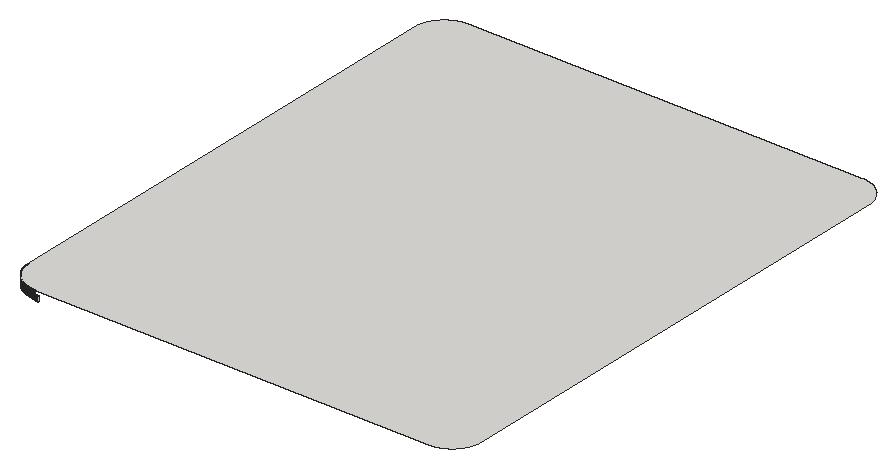
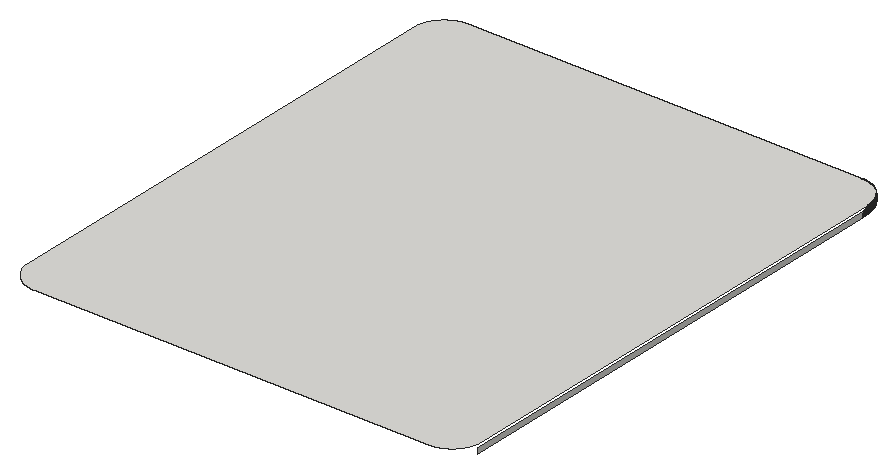
# SketchUp Ruby script. Lengths in inches.
U = 1.inch
M = Sketchup.active_model
def pt(a) = Geom::Point3d.new(a.map { |v| v * U })
def face(e, loops, mat)
  f = e.add_face(loops[0].map { |a| pt(a) })
  loops[1..].each { |l| e.add_face(l.map { |a| pt(a) }).erase! }
  f.material = f.back_material = mat if mat
  f
end
# faces: each face lists its corners as indices into pts; further lists are holes
def faces(e, pts, list, mat = nil) = list.each { |f| face(e, (f[0].is_a?(Array) ? f : [f]).map { |l| l.map { |i| pts[i] } }, mat) }
# xy, xz, yz: faces in a plane at the given z, y or x. An outline is a flat list of corners, or four numbers for a rectangle; further outlines are holes
def ring(l) = l.size == 4 ? [[l[0], l[1]], [l[2], l[1]], [l[2], l[3]], [l[0], l[3]]] : l.each_slice(2).to_a
def flat(e, list, mat, &to3) = list.each { |f| face(e, (f[0].is_a?(Array) ? f : [f]).map { |l| ring(l).map { |u, v| to3.(u, v) } }, mat) }
def xy(e, z, list, mat = nil) = flat(e, list, mat) { |x, y| [x, y, z] }
def xz(e, y, list, mat = nil) = flat(e, list, mat) { |x, z| [x, y, z] }
def yz(e, x, list, mat = nil) = flat(e, list, mat) { |y, z| [x, y, z] }
def lines(e, pts, list) = list.each { |a, b| e.add_line(pt(pts[a]), pt(pts[b])) }
# prism: a flat outline (further loops are holes) pulled along v
def prism(e, loops, v, mat = nil)
  f = face(e, loops, mat); d = Geom::Vector3d.new(v.map { |x| x * U })
  f.pushpull(f.normal.samedirection?(d) ? d.length : -d.length)
end
def box(e, o, s, mat = nil) = prism(e, [[o, [o[0] + s[0], o[1], o[2]], [o[0] + s[0], o[1] + s[1], o[2]], [o[0], o[1] + s[1], o[2]]]], [0, 0, s[2]], mat)
def at(x, y, z, deg = 0) = Geom::Transformation.translation(pt([x, y, z])) * Geom::Transformation.rotation(ORIGIN, Z_AXIS, deg.degrees)
def axes(o, x, y, z) = Geom::Transformation.new([*x, 0, *y, 0, *z, 0, *pt(o).to_a, 1])
def part(name) = M.definitions.add(name)
# library, detail: a bought-in or finely detailed component or shape, given as its bounding box
def library(name, o, s) = part(name).tap { |d| box(d.entities, o, s) }
def detail(e, o, s) = box(e.add_group.entities, o, s)
def put(e, d, t, mat = nil) = e.add_instance(d, t).tap { |i| i.material = mat if mat }
def group(e, t, mat = nil) = e.add_group.tap { |g| g.transformation = t; g.material = mat if mat }.entities
root = M.entities
M.materials.add("[Formica Graystone]").color = [224, 223, 219]
xy(root,427.82,[[17.6875,229,174.3125,229,174.47,229.01,174.63,229.02,174.78,229.03,175.1,229.05,175.25,229.07,175.41,229.08,175.57,229.1,175.72,229.125,175.88,229.15,176.03,229.17,176.1875,229.2,176.34,229.23,176.49,229.26,176.65,229.3,176.8,229.33,176.95,229.37,177.11,229.41,177.41,229.49,177.86,229.64,178.01,229.6875,178.15,229.74,178.3,229.8,178.45,229.85,178.59,229.91,178.74,229.97,178.88,230.04,179.02,230.1,179.17,230.17,179.73,230.45,179.86,230.53,180,230.61,180.14,230.6875,180.27,230.77,180.4,230.85,180.54,230.9375,180.67,231.02,180.93,231.2,181.05,231.29,181.18,231.38,181.31,231.48,181.43,231.58,181.55,231.67,181.67,231.77,181.91,231.98,182.03,232.08,182.15,232.1875,182.26,232.3,182.375,232.4,182.49,232.51,182.6,232.625,182.7,232.74,182.8125,232.85,182.92,232.97,183.02,233.09,183.23,233.33,183.33,233.45,183.42,233.57,183.52,233.69,183.62,233.82,183.71,233.95,183.8,234.07,183.98,234.33,184.0625,234.46,184.15,234.6,184.23,234.73,184.3125,234.86,184.39,235,184.47,235.14,184.55,235.27,184.83,235.83,184.9,235.98,184.96,236.12,185.03,236.26,185.09,236.41,185.15,236.55,185.2,236.7,185.26,236.85,185.3125,236.99,185.36,237.14,185.51,237.59,185.59,237.89,185.63,238.05,185.67,238.2,185.7,238.35,185.74,238.51,185.77,238.66,185.8,238.8125,185.83,238.97,185.85,239.12,185.875,239.28,185.9,239.43,185.92,239.59,185.93,239.75,185.95,239.9,185.97,240.22,185.98,240.37,185.99,240.53,186,240.6875,186,432.3125,185.99,432.47,185.98,432.63,185.97,432.78,185.95,433.1,185.93,433.25,185.92,433.41,185.9,433.57,185.875,433.72,185.85,433.88,185.83,434.03,185.8,434.1875,185.77,434.34,185.74,434.49,185.7,434.65,185.67,434.8,185.63,434.95,185.59,435.11,185.51,435.41,185.36,435.86,185.3125,436.01,185.26,436.15,185.2,436.3,185.15,436.45,185.09,436.59,185.03,436.74,184.96,436.88,184.9,437.02,184.83,437.17,184.55,437.73,184.47,437.86,184.39,438,184.3125,438.14,184.23,438.27,184.15,438.4,184.0625,438.54,183.98,438.67,183.8,438.93,183.71,439.05,183.62,439.18,183.52,439.31,183.42,439.43,183.33,439.55,183.23,439.67,183.02,439.91,182.92,440.03,182.8125,440.15,182.7,440.26,182.6,440.375,182.49,440.49,182.375,440.6,182.26,440.7,182.15,440.8125,182.03,440.92,181.91,441.02,181.67,441.23,181.55,441.33,181.43,441.42,181.31,441.52,181.18,441.62,181.05,441.71,180.93,441.8,180.67,441.98,180.54,442.0625,180.4,442.15,180.27,442.23,180.14,442.3125,180,442.39,179.86,442.47,179.73,442.55,179.17,442.83,179.02,442.9,178.88,442.96,178.74,443.03,178.59,443.09,178.45,443.15,178.3,443.2,178.15,443.26,178.01,443.3125,177.86,443.36,177.41,443.51,177.11,443.59,176.95,443.63,176.8,443.67,176.65,443.7,176.49,443.74,176.34,443.77,176.1875,443.8,176.03,443.83,175.88,443.85,175.72,443.875,175.57,443.9,175.41,443.92,175.25,443.93,175.1,443.95,174.78,443.97,174.63,443.98,174.47,443.99,174.3125,444,17.6875,444,17.53,443.99,17.37,443.98,17.22,443.97,16.9,443.95,16.75,443.93,16.59,443.92,16.43,443.9,16.28,443.875,16.12,443.85,15.97,443.83,15.8125,443.8,15.66,443.77,15.51,443.74,15.35,443.7,15.2,443.67,15.05,443.63,14.89,443.59,14.59,443.51,14.14,443.36,13.99,443.3125,13.85,443.26,13.7,443.2,13.55,443.15,13.41,443.09,13.26,443.03,13.12,442.96,12.98,442.9,12.83,442.83,12.27,442.55,12.14,442.47,12,442.39,11.86,442.3125,11.73,442.23,11.6,442.15,11.46,442.0625,11.33,441.98,11.07,441.8,10.95,441.71,10.82,441.62,10.69,441.52,10.57,441.42,10.45,441.33,10.33,441.23,10.09,441.02,9.97,440.92,9.85,440.8125,9.74,440.7,9.625,440.6,9.51,440.49,9.4,440.375,9.3,440.26,9.1875,440.15,9.08,440.03,8.98,439.91,8.77,439.67,8.67,439.55,8.58,439.43,8.48,439.31,8.38,439.18,8.29,439.05,8.2,438.93,8.02,438.67,7.9375,438.54,7.85,438.4,7.77,438.27,7.6875,438.14,7.61,438,7.53,437.86,7.45,437.73,7.17,437.17,7.1,437.02,7.04,436.88,6.97,436.74,6.91,436.59,6.85,436.45,6.8,436.3,6.74,436.15,6.6875,436.01,6.64,435.86,6.49,435.41,6.41,435.11,6.37,434.95,6.33,434.8,6.3,434.65,6.26,434.49,6.23,434.34,6.2,434.1875,6.17,434.03,6.15,433.88,6.125,433.72,6.1,433.57,6.08,433.41,6.07,433.25,6.05,433.1,6.03,432.78,6.02,432.63,6.01,432.47,6,432.3125,6,240.6875,6.01,240.53,6.02,240.37,6.03,240.22,6.05,239.9,6.07,239.75,6.08,239.59,6.1,239.43,6.125,239.28,6.15,239.12,6.17,238.97,6.2,238.8125,6.23,238.66,6.26,238.51,6.3,238.35,6.33,238.2,6.37,238.05,6.41,237.89,6.49,237.59,6.64,237.14,6.6875,236.99,6.74,236.85,6.8,236.7,6.85,236.55,6.91,236.41,6.97,236.26,7.04,236.12,7.1,235.98,7.17,235.83,7.45,235.27,7.53,235.14,7.61,235,7.6875,234.86,7.77,234.73,7.85,234.6,7.9375,234.46,8.02,234.33,8.2,234.07,8.29,233.95,8.38,233.82,8.48,233.69,8.58,233.57,8.67,233.45,8.77,233.33,8.98,233.09,9.08,232.97,9.1875,232.85,9.3,232.74,9.4,232.625,9.51,232.51,9.625,232.4,9.74,232.3,9.85,232.1875,9.97,232.08,10.09,231.98,10.33,231.77,10.45,231.67,10.57,231.58,10.69,231.48,10.82,231.38,10.95,231.29,11.07,231.2,11.33,231.02,11.46,230.9375,11.6,230.85,11.73,230.77,11.86,230.6875,12,230.61,12.14,230.53,12.27,230.45,12.83,230.17,12.98,230.1,13.12,230.04,13.26,229.97,13.41,229.91,13.55,229.85,13.7,229.8,13.85,229.74,13.99,229.6875,14.14,229.64,14.59,229.49,14.89,229.41,15.05,229.37,15.2,229.33,15.35,229.3,15.51,229.26,15.66,229.23,15.8125,229.2,15.97,229.17,16.12,229.15,16.28,229.125,16.43,229.1,16.59,229.08,16.75,229.07,16.9,229.05,17.22,229.03,17.37,229.02,17.53,229.01]],"[Formica Graystone]")
xz(root,229,[[17.6875,424.82,17.84,427.82],[17.84,424.82,18,427.82]],"[Formica Graystone]")
xz(root,231,[[17.74,422.82,17.87,424.82],[17.87,422.82,18,424.82]],"[Formica Graystone]")
xz(root,231.01,[[17.48,422.82,17.61,424.82]],"[Formica Graystone]")
yz(root,6,[[240.6875,424.82,240.84,427.82],[240.84,424.82,241,427.82]],"[Formica Graystone]")
yz(root,8,[[240.74,422.82,240.87,424.82],[240.87,422.82,241,424.82],[241,422.82,432,424.82]],"[Formica Graystone]")
yz(root,8.01,[[240.48,422.82,240.61,424.82]],"[Formica Graystone]")
p = [[17.08,231.04,422.82],[17.08,231.04,424.82],[16.95,231.05,424.82],[16.95,231.05,422.82],[17.22,231.03,422.82],[17.22,231.03,424.82],
  [17.35,231.02,422.82],[17.35,231.02,424.82],[17.48,231.01,422.82],[17.48,231.01,424.82],[17.74,231,422.82],[17.74,231,424.82],
  [17.61,231.01,424.82],[17.61,231.01,422.82],[16.31,231.14,422.82],[16.31,231.14,424.82],[16.18,231.17,424.82],[16.18,231.17,422.82],
  [16.4375,231.125,422.82],[16.4375,231.125,424.82],[16.57,231.1,422.82],[16.57,231.1,424.82],[16.69,231.09,422.82],[16.69,231.09,424.82],
  [16.82,231.07,422.82],[16.82,231.07,424.82],[15.79,231.25,422.82],[15.79,231.25,424.82],[15.67,231.28,424.82],[15.67,231.28,422.82],
  [15.92,231.22,422.82],[15.92,231.22,424.82],[16.05,231.19,422.82],[16.05,231.19,424.82],[15.41,231.34,422.82],[15.41,231.34,424.82],
  [15.29,231.375,424.82],[15.29,231.375,422.82],[15.54,231.31,422.82],[15.54,231.31,424.82],[15.03,231.45,422.82],[15.03,231.45,424.82],
  [14.91,231.49,424.82],[14.91,231.49,422.82],[15.16,231.41,422.82],[15.16,231.41,424.82],[14.79,231.53,422.82],[14.79,231.53,424.82],
  [14.66,231.57,424.82],[14.66,231.57,422.82],[14.54,231.62,422.82],[14.54,231.62,424.82],[14.42,231.66,424.82],[14.42,231.66,422.82],
  [14.29,231.71,422.82],[14.29,231.71,424.82],[14.17,231.76,424.82],[14.17,231.76,422.82],[14.05,231.8125,422.82],[14.05,231.8125,424.82],
  [13.93,231.86,424.82],[13.93,231.86,422.82],[13.8125,231.92,422.82],[13.8125,231.92,424.82],[13.69,231.97,424.82],[13.69,231.97,422.82],
  [13.58,232.03,422.82],[13.58,232.03,424.82],[13.46,232.09,424.82],[13.46,232.09,422.82],[13.34,232.15,424.82],[13.34,232.15,422.82],
  [13.23,232.21,422.82],[13.23,232.21,424.82],[13.11,232.28,424.82],[13.11,232.28,422.82],[13,232.34,422.82],[13,232.34,424.82],
  [12.89,232.41,424.82],[12.89,232.41,422.82],[12.78,232.47,424.82],[12.78,232.47,422.82],[12.66,232.54,422.82],[12.66,232.54,424.82],
  [12.55,232.61,424.82],[12.55,232.61,422.82],[12.44,232.69,424.82],[12.44,232.69,422.82],[12.34,232.76,424.82],[12.34,232.76,422.82],
  [12.23,232.83,422.82],[12.23,232.83,424.82],[12.12,232.91,424.82],[12.12,232.91,422.82],[12.02,232.99,424.82],[12.02,232.99,422.82],
  [11.91,233.07,424.82],[11.91,233.07,422.82],[11.81,233.15,422.82],[11.81,233.15,424.82],[11.71,233.23,424.82],[11.71,233.23,422.82],
  [11.61,233.3125,424.82],[11.61,233.3125,422.82],[11.51,233.4,424.82],[11.51,233.4,422.82],[11.41,233.48,424.82],[11.41,233.48,422.82],
  [11.31,233.57,424.82],[11.31,233.57,422.82],[11.21,233.66,424.82],[11.21,233.66,422.82],[11.12,233.75,422.82],[11.12,233.75,424.82],
  [11.02,233.84,424.82],[11.02,233.84,422.82],[10.93,233.93,424.82],[10.93,233.93,422.82],[10.84,234.02,424.82],[10.84,234.02,422.82],
  [10.75,234.12,424.82],[10.75,234.12,422.82],[10.66,234.21,424.82],[10.66,234.21,422.82],[10.57,234.31,424.82],[10.57,234.31,422.82],
  [10.48,234.41,424.82],[10.48,234.41,422.82],[10.4,234.51,424.82],[10.4,234.51,422.82],[10.3125,234.61,424.82],[10.3125,234.61,422.82],
  [10.23,234.71,424.82],[10.23,234.71,422.82],[10.15,234.81,424.82],[10.15,234.81,422.82],[10.07,234.91,424.82],[10.07,234.91,422.82],
  [9.99,235.02,424.82],[9.99,235.02,422.82],[9.91,235.12,424.82],[9.91,235.12,422.82],[9.83,235.23,424.82],[9.83,235.23,422.82],
  [9.76,235.34,424.82],[9.76,235.34,422.82],[9.69,235.44,424.82],[9.69,235.44,422.82],[9.61,235.55,424.82],[9.61,235.55,422.82],
  [9.54,235.66,424.82],[9.54,235.66,422.82],[9.47,235.78,424.82],[9.47,235.78,422.82],[9.41,235.89,424.82],[9.41,235.89,422.82],
  [9.34,236,424.82],[9.34,236,422.82],[9.28,236.11,424.82],[9.28,236.11,422.82],[9.21,236.23,424.82],[9.21,236.23,422.82],
  [9.15,236.34,424.82],[9.15,236.34,422.82],[9.09,236.46,424.82],[9.09,236.46,422.82],[9.03,236.58,424.82],[9.03,236.58,422.82],
  [8.97,236.69,424.82],[8.97,236.69,422.82],[8.92,236.8125,424.82],[8.92,236.8125,422.82],[8.86,236.93,424.82],[8.86,236.93,422.82],
  [8.8125,237.05,424.82],[8.8125,237.05,422.82],[8.76,237.17,424.82],[8.76,237.17,422.82],[8.71,237.29,424.82],[8.71,237.29,422.82],
  [8.66,237.42,424.82],[8.66,237.42,422.82],[8.62,237.54,424.82],[8.62,237.54,422.82],[8.57,237.66,424.82],[8.57,237.66,422.82],
  [8.53,237.79,424.82],[8.53,237.79,422.82],[8.49,237.91,424.82],[8.49,237.91,422.82],[8.45,238.03,424.82],[8.45,238.03,422.82],
  [8.41,238.16,424.82],[8.41,238.16,422.82],[8.375,238.29,424.82],[8.375,238.29,422.82],[8.34,238.41,424.82],[8.34,238.41,422.82],
  [8.31,238.54,424.82],[8.31,238.54,422.82],[8.28,238.67,424.82],[8.28,238.67,422.82],[8.25,238.79,424.82],[8.25,238.79,422.82],
  [8.22,238.92,424.82],[8.22,238.92,422.82],[8.19,239.05,424.82],[8.19,239.05,422.82],[8.17,239.18,424.82],[8.17,239.18,422.82],
  [8.14,239.31,424.82],[8.14,239.31,422.82],[8.125,239.4375,424.82],[8.125,239.4375,422.82],[8.1,239.57,424.82],[8.1,239.57,422.82],
  [8.09,239.69,424.82],[8.09,239.69,422.82],[8.07,239.82,424.82],[8.07,239.82,422.82],[8.05,239.95,424.82],[8.05,239.95,422.82],
  [8.04,240.08,424.82],[8.04,240.08,422.82],[8.03,240.22,424.82],[8.03,240.22,422.82],[8.02,240.35,424.82],[8.02,240.35,422.82],
  [8.01,240.48,424.82],[8.01,240.48,422.82],[8.01,240.61,422.82],[8.01,240.61,424.82],[8,240.74,424.82],[8,240.74,422.82],
  [16.9,229.05,424.82],[17.06,229.04,424.82],[17.06,229.04,427.82],[16.9,229.05,427.82],[17.22,229.03,424.82],[17.22,229.03,427.82],
  [17.37,229.02,424.82],[17.37,229.02,427.82],[17.53,229.01,424.82],[17.53,229.01,427.82],[17.6875,229,424.82],[17.6875,229,427.82],
  [15.97,229.17,424.82],[16.12,229.15,424.82],[16.12,229.15,427.82],[15.97,229.17,427.82],[16.28,229.125,424.82],[16.28,229.125,427.82],
  [16.43,229.1,424.82],[16.43,229.1,427.82],[16.59,229.08,424.82],[16.59,229.08,427.82],[16.75,229.07,424.82],[16.75,229.07,427.82],
  [15.51,229.26,424.82],[15.66,229.23,424.82],[15.66,229.23,427.82],[15.51,229.26,427.82],[15.8125,229.2,424.82],[15.8125,229.2,427.82],
  [15.05,229.37,424.82],[15.2,229.33,424.82],[15.2,229.33,427.82],[15.05,229.37,427.82],[15.35,229.3,424.82],[15.35,229.3,427.82],
  [14.74,229.45,424.82],[14.89,229.41,424.82],[14.89,229.41,427.82],[14.74,229.45,427.82],[14.29,229.59,424.82],[14.44,229.54,424.82],
  [14.44,229.54,427.82],[14.29,229.59,427.82],[14.59,229.49,424.82],[14.59,229.49,427.82],[13.99,229.6875,424.82],[14.14,229.64,424.82],
  [14.14,229.64,427.82],[13.99,229.6875,427.82],[13.7,229.8,424.82],[13.85,229.74,424.82],[13.85,229.74,427.82],[13.7,229.8,427.82],
  [13.55,229.85,424.82],[13.55,229.85,427.82],[13.26,229.97,424.82],[13.41,229.91,424.82],[13.41,229.91,427.82],[13.26,229.97,427.82],
  [12.98,230.1,424.82],[13.12,230.04,424.82],[13.12,230.04,427.82],[12.98,230.1,427.82],[12.83,230.17,424.82],[12.83,230.17,427.82],
  [12.55,230.31,424.82],[12.69,230.24,424.82],[12.69,230.24,427.82],[12.55,230.31,427.82],[12.41,230.38,424.82],[12.41,230.38,427.82],
  [12.27,230.45,424.82],[12.27,230.45,427.82],[12,230.61,424.82],[12.14,230.53,424.82],[12.14,230.53,427.82],[12,230.61,427.82],
  [11.86,230.6875,424.82],[11.86,230.6875,427.82],[11.73,230.77,424.82],[11.73,230.77,427.82],[11.6,230.85,424.82],[11.6,230.85,427.82],
  [11.33,231.02,424.82],[11.46,230.9375,424.82],[11.46,230.9375,427.82],[11.33,231.02,427.82],[11.2,231.11,424.82],[11.2,231.11,427.82],
  [11.07,231.2,424.82],[11.07,231.2,427.82],[10.95,231.29,424.82],[10.95,231.29,427.82],[10.82,231.38,424.82],[10.82,231.38,427.82],
  [10.69,231.48,424.82],[10.69,231.48,427.82],[10.57,231.58,424.82],[10.57,231.58,427.82],[10.45,231.67,424.82],[10.45,231.67,427.82],
  [10.33,231.77,424.82],[10.33,231.77,427.82],[10.21,231.875,424.82],[10.21,231.875,427.82],[10.09,231.98,424.82],[10.09,231.98,427.82],
  [9.97,232.08,424.82],[9.97,232.08,427.82],[9.85,232.1875,424.82],[9.85,232.1875,427.82],[9.74,232.3,424.82],[9.74,232.3,427.82],
  [9.625,232.4,424.82],[9.625,232.4,427.82],[9.51,232.51,424.82],[9.51,232.51,427.82],[9.4,232.625,424.82],[9.4,232.625,427.82],
  [9.3,232.74,424.82],[9.3,232.74,427.82],[9.1875,232.85,424.82],[9.1875,232.85,427.82],[9.08,232.97,424.82],[9.08,232.97,427.82],
  [8.98,233.09,424.82],[8.98,233.09,427.82],[8.875,233.21,424.82],[8.875,233.21,427.82],[8.77,233.33,424.82],[8.77,233.33,427.82],
  [8.67,233.45,424.82],[8.67,233.45,427.82],[8.58,233.57,424.82],[8.58,233.57,427.82],[8.48,233.69,424.82],[8.48,233.69,427.82],
  [8.38,233.82,424.82],[8.38,233.82,427.82],[8.29,233.95,424.82],[8.29,233.95,427.82],[8.2,234.07,424.82],[8.2,234.07,427.82],
  [8.11,234.2,424.82],[8.11,234.2,427.82],[8.02,234.33,424.82],[8.02,234.33,427.82],[7.9375,234.46,424.82],[7.9375,234.46,427.82],
  [7.85,234.6,424.82],[7.85,234.6,427.82],[7.77,234.73,424.82],[7.77,234.73,427.82],[7.6875,234.86,424.82],[7.6875,234.86,427.82],
  [7.61,235,424.82],[7.61,235,427.82],[7.53,235.14,424.82],[7.53,235.14,427.82],[7.45,235.27,424.82],[7.45,235.27,427.82],
  [7.38,235.41,424.82],[7.38,235.41,427.82],[7.31,235.55,424.82],[7.31,235.55,427.82],[7.24,235.69,424.82],[7.24,235.69,427.82],
  [7.17,235.83,424.82],[7.17,235.83,427.82],[7.1,235.98,424.82],[7.1,235.98,427.82],[7.04,236.12,424.82],[7.04,236.12,427.82],
  [6.97,236.26,424.82],[6.97,236.26,427.82],[6.91,236.41,424.82],[6.91,236.41,427.82],[6.85,236.55,424.82],[6.85,236.55,427.82],
  [6.8,236.7,424.82],[6.8,236.7,427.82],[6.74,236.85,424.82],[6.74,236.85,427.82],[6.6875,236.99,424.82],[6.6875,236.99,427.82],
  [6.64,237.14,424.82],[6.64,237.14,427.82],[6.59,237.29,424.82],[6.59,237.29,427.82],[6.54,237.44,424.82],[6.54,237.44,427.82],
  [6.49,237.59,424.82],[6.49,237.59,427.82],[6.45,237.74,424.82],[6.45,237.74,427.82],[6.41,237.89,424.82],[6.41,237.89,427.82],
  [6.37,238.05,424.82],[6.37,238.05,427.82],[6.33,238.2,424.82],[6.33,238.2,427.82],[6.3,238.35,424.82],[6.3,238.35,427.82],
  [6.26,238.51,424.82],[6.26,238.51,427.82],[6.23,238.66,424.82],[6.23,238.66,427.82],[6.2,238.8125,424.82],[6.2,238.8125,427.82],
  [6.17,238.97,424.82],[6.17,238.97,427.82],[6.15,239.12,424.82],[6.15,239.12,427.82],[6.125,239.28,424.82],[6.125,239.28,427.82],
  [6.1,239.43,424.82],[6.1,239.43,427.82],[6.08,239.59,424.82],[6.08,239.59,427.82],[6.07,239.75,424.82],[6.07,239.75,427.82],
  [6.05,239.9,424.82],[6.05,239.9,427.82],[6.04,240.06,424.82],[6.04,240.06,427.82],[6.03,240.22,424.82],[6.03,240.22,427.82],
  [6.02,240.37,424.82],[6.02,240.37,427.82],[6.01,240.53,424.82],[6.01,240.53,427.82],[6,240.6875,424.82],[6,240.6875,427.82]]
faces(root,p,[[0,1,2,3],[4,5,1,0],[6,7,5,4],[8,9,7,6],[10,11,12,13],[14,15,16,17],[18,19,15,14],[20,21,19,18],
  [22,23,21,20],[24,25,23,22],[3,2,25,24],[26,27,28,29],[30,31,27,26],[32,33,31,30],[17,16,33,32],[34,35,36,37],
  [38,39,35,34],[29,28,39,38],[40,41,42,43],[44,45,41,40],[37,36,45,44],[46,47,48,49],[43,42,47,46],[50,51,52,53],
  [49,48,51,50],[54,55,56,57],[53,52,55,54],[58,59,60,61],[57,56,59,58],[62,63,64,65],[61,60,63,62],[66,67,68,69],
  [65,64,67,66],[69,68,70,71],[72,73,74,75],[71,70,73,72],[76,77,78,79],[75,74,77,76],[79,78,80,81],[82,83,84,85],
  [81,80,83,82],[85,84,86,87],[87,86,88,89],[90,91,92,93],[89,88,91,90],[93,92,94,95],[95,94,96,97],[98,99,100,101],
  [97,96,99,98],[101,100,102,103],[103,102,104,105],[105,104,106,107],[107,106,108,109],[109,108,110,111],[112,113,114,115],[111,110,113,112],
  [115,114,116,117],[117,116,118,119],[119,118,120,121],[121,120,122,123],[123,122,124,125],[125,124,126,127],[127,126,128,129],[129,128,130,131],
  [131,130,132,133],[133,132,134,135],[135,134,136,137],[137,136,138,139],[139,138,140,141],[141,140,142,143],[143,142,144,145],[145,144,146,147],
  [147,146,148,149],[149,148,150,151],[151,150,152,153],[153,152,154,155],[155,154,156,157],[157,156,158,159],[159,158,160,161],[161,160,162,163],
  [163,162,164,165],[165,164,166,167],[167,166,168,169],[169,168,170,171],[171,170,172,173],[173,172,174,175],[175,174,176,177],[177,176,178,179],
  [179,178,180,181],[181,180,182,183],[183,182,184,185],[185,184,186,187],[187,186,188,189],[189,188,190,191],[191,190,192,193],[193,192,194,195],
  [195,194,196,197],[197,196,198,199],[199,198,200,201],[201,200,202,203],[203,202,204,205],[205,204,206,207],[207,206,208,209],[209,208,210,211],
  [211,210,212,213],[213,212,214,215],[215,214,216,217],[217,216,218,219],[219,218,220,221],[221,220,222,223],[223,222,224,225],[225,224,226,227],
  [227,226,228,229],[230,231,232,233],[234,235,236,237],[235,238,239,236],[238,240,241,239],[240,242,243,241],[242,244,245,243],[246,247,248,249],
  [247,250,251,248],[250,252,253,251],[252,254,255,253],[254,256,257,255],[256,234,237,257],[258,259,260,261],[259,262,263,260],[262,246,249,263],
  [264,265,266,267],[265,268,269,266],[268,258,261,269],[270,271,272,273],[271,264,267,272],[274,275,276,277],[275,278,279,276],[278,270,273,279],
  [280,281,282,283],[281,274,277,282],[284,285,286,287],[285,280,283,286],[288,284,287,289],[290,291,292,293],[291,288,289,292],[294,295,296,297],
  [295,290,293,296],[298,294,297,299],[300,301,302,303],[301,298,299,302],[304,300,303,305],[306,304,305,307],[308,309,310,311],[309,306,307,310],
  [312,308,311,313],[314,312,313,315],[316,314,315,317],[318,319,320,321],[319,316,317,320],[322,318,321,323],[324,322,323,325],[326,324,325,327],
  [328,326,327,329],[330,328,329,331],[332,330,331,333],[334,332,333,335],[336,334,335,337],[338,336,337,339],[340,338,339,341],[342,340,341,343],
  [344,342,343,345],[346,344,345,347],[348,346,347,349],[350,348,349,351],[352,350,351,353],[354,352,353,355],[356,354,355,357],[358,356,357,359],
  [360,358,359,361],[362,360,361,363],[364,362,363,365],[366,364,365,367],[368,366,367,369],[370,368,369,371],[372,370,371,373],[374,372,373,375],
  [376,374,375,377],[378,376,377,379],[380,378,379,381],[382,380,381,383],[384,382,383,385],[386,384,385,387],[388,386,387,389],[390,388,389,391],
  [392,390,391,393],[394,392,393,395],[396,394,395,397],[398,396,397,399],[400,398,399,401],[402,400,401,403],[404,402,403,405],[406,404,405,407],
  [408,406,407,409],[410,408,409,411],[412,410,411,413],[414,412,413,415],[416,414,415,417],[418,416,417,419],[420,418,419,421],[422,420,421,423],
  [424,422,423,425],[426,424,425,427],[428,426,427,429],[430,428,429,431],[432,430,431,433],[434,432,433,435],[436,434,435,437],[438,436,437,439],
  [440,438,439,441],[442,440,441,443],[444,442,443,445],[446,444,445,447],[448,446,447,449],[450,448,449,451],[452,450,451,453],[454,452,453,455],
  [456,454,455,457],[458,456,457,459],[460,458,459,461],[462,460,461,463],[464,462,463,465],[466,464,465,467]],"[Formica Graystone]")
